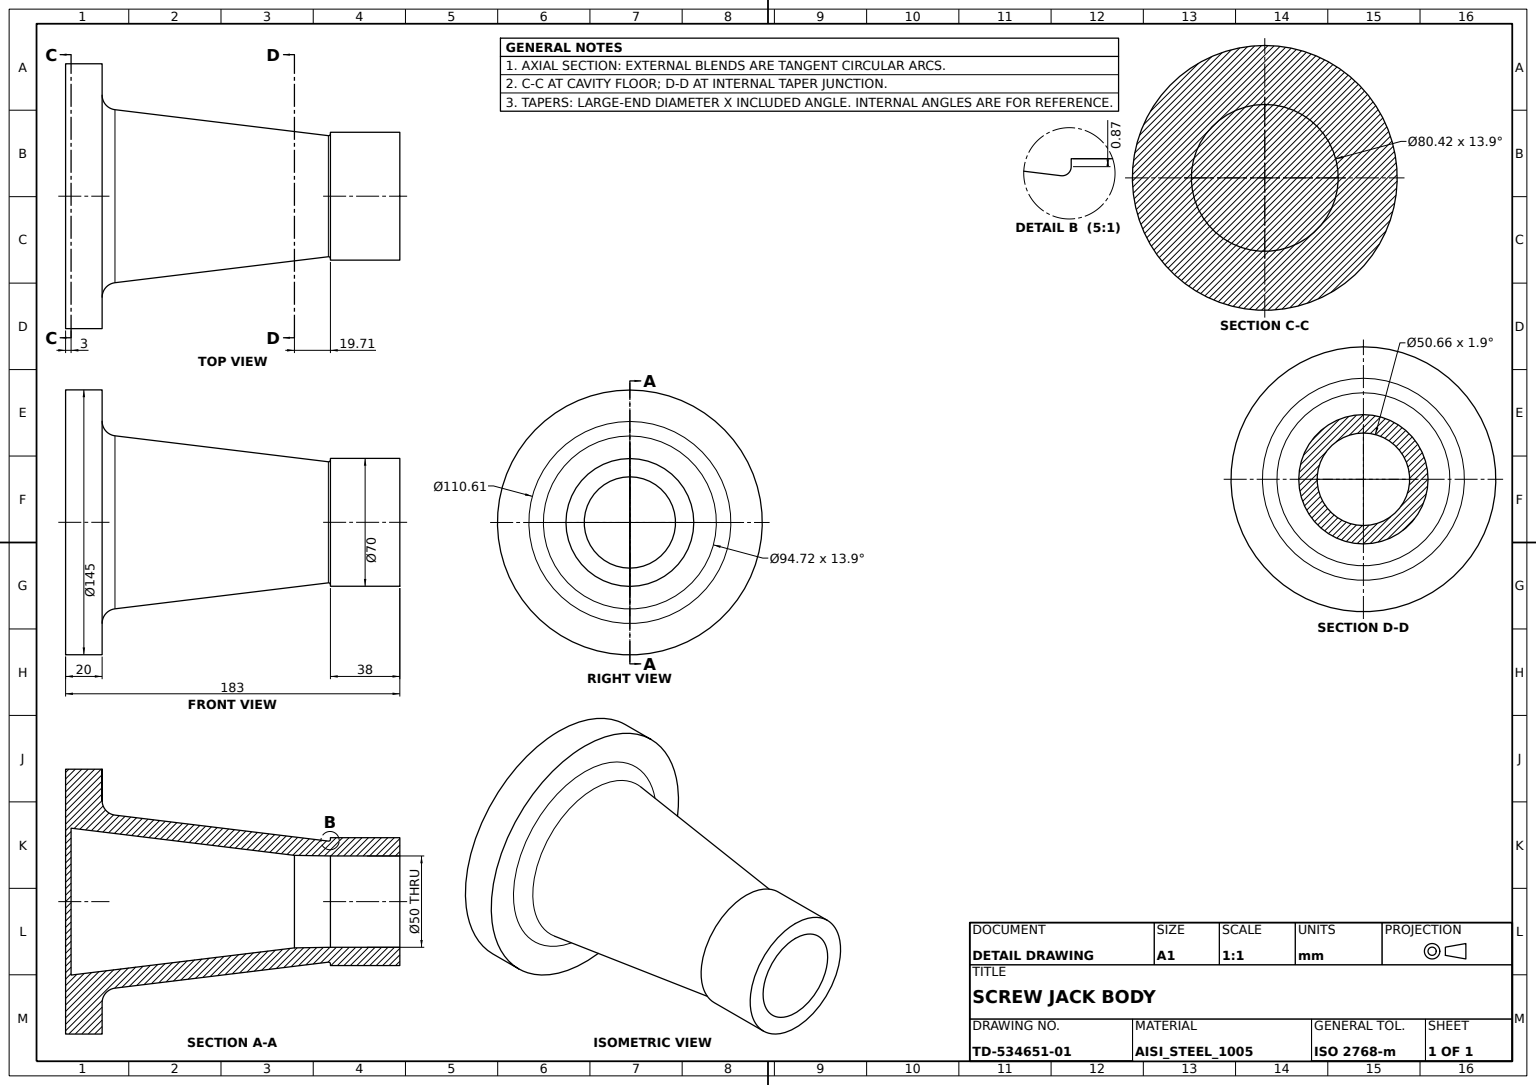
ISO-10303-21;
HEADER;
FILE_DESCRIPTION((''),'2;1');
FILE_NAME('','',(''),(''),'','','');
FILE_SCHEMA(('AUTOMOTIVE_DESIGN'));
ENDSEC;
DATA;
#1=APPLICATION_CONTEXT('');
#2=PRODUCT_CONTEXT('',#1,'mechanical');
#3=PRODUCT('','','',(#2));
#4=PRODUCT_DEFINITION_FORMATION('','',#3);
#5=PRODUCT_DEFINITION_CONTEXT('',#1,'design');
#6=PRODUCT_DEFINITION('','',#4,#5);
#7=PRODUCT_DEFINITION_SHAPE('','',#6);
#8=(LENGTH_UNIT()NAMED_UNIT(*)SI_UNIT(.MILLI.,.METRE.));
#9=(NAMED_UNIT(*)PLANE_ANGLE_UNIT()SI_UNIT($,.RADIAN.));
#10=(NAMED_UNIT(*)SI_UNIT($,.STERADIAN.)SOLID_ANGLE_UNIT());
#11=UNCERTAINTY_MEASURE_WITH_UNIT(LENGTH_MEASURE(0.005),#8,'distance_accuracy_value','');
#12=(GEOMETRIC_REPRESENTATION_CONTEXT(3)GLOBAL_UNCERTAINTY_ASSIGNED_CONTEXT((#11))GLOBAL_UNIT_ASSIGNED_CONTEXT((#8,#9,#10))REPRESENTATION_CONTEXT('',''));
#13=CARTESIAN_POINT('',(-35.,0.,183.));
#14=VERTEX_POINT('',#13);
#15=CARTESIAN_POINT('',(0.,0.,183.));
#16=DIRECTION('',(0.,0.,-1.));
#17=DIRECTION('',(-1.,0.,0.));
#18=AXIS2_PLACEMENT_3D('',#15,#16,#17);
#19=CIRCLE('',#18,35.);
#20=EDGE_CURVE('',#14,#14,#19,.T.);
#21=ORIENTED_EDGE('',*,*,#20,.F.);
#22=EDGE_LOOP('',(#21));
#23=FACE_BOUND('',#22,.T.);
#24=CARTESIAN_POINT('',(-25.,0.,183.));
#25=VERTEX_POINT('',#24);
#26=CIRCLE('',#18,25.);
#27=EDGE_CURVE('',#25,#25,#26,.T.);
#28=ORIENTED_EDGE('',*,*,#27,.T.);
#29=EDGE_LOOP('',(#28));
#30=FACE_BOUND('',#29,.T.);
#31=AXIS2_PLACEMENT_3D('',#24,#16,#17);
#32=PLANE('',#31);
#33=ADVANCED_FACE('',(#23,#30),#32,.F.);
#34=CARTESIAN_POINT('',(-33.136466,0.,143.879141));
#35=VERTEX_POINT('',#34);
#36=CARTESIAN_POINT('',(0.,0.,143.879141));
#37=AXIS2_PLACEMENT_3D('',#36,#16,#17);
#38=CIRCLE('',#37,33.136466);
#39=EDGE_CURVE('',#35,#35,#38,.T.);
#40=ORIENTED_EDGE('',*,*,#39,.F.);
#41=EDGE_LOOP('',(#40));
#42=FACE_BOUND('',#41,.T.);
#43=CARTESIAN_POINT('',(-34.129136,0.,145.));
#44=VERTEX_POINT('',#43);
#45=CARTESIAN_POINT('',(0.,0.,145.));
#46=AXIS2_PLACEMENT_3D('',#45,#16,#17);
#47=CIRCLE('',#46,34.129136);
#48=EDGE_CURVE('',#44,#44,#47,.T.);
#49=ORIENTED_EDGE('',*,*,#48,.T.);
#50=EDGE_LOOP('',(#49));
#51=FACE_BOUND('',#50,.T.);
#52=CARTESIAN_POINT('',(0.,0.,144.));
#53=AXIS2_PLACEMENT_3D('',#52,#16,#17);
#54=TOROIDAL_SURFACE('',#53,34.129136,1.);
#55=ADVANCED_FACE('',(#42,#51),#54,.F.);
#56=ORIENTED_EDGE('',*,*,#27,.F.);
#57=EDGE_LOOP('',(#56));
#58=FACE_BOUND('',#57,.T.);
#59=CARTESIAN_POINT('',(-25.,0.,145.));
#60=VERTEX_POINT('',#59);
#61=CIRCLE('',#46,25.);
#62=EDGE_CURVE('',#60,#60,#61,.T.);
#63=ORIENTED_EDGE('',*,*,#62,.T.);
#64=EDGE_LOOP('',(#63));
#65=FACE_BOUND('',#64,.T.);
#66=CARTESIAN_POINT('',(0.,0.,0.));
#67=AXIS2_PLACEMENT_3D('',#66,#16,#17);
#68=CYLINDRICAL_SURFACE('',#67,25.);
#69=ADVANCED_FACE('',(#58,#65),#68,.F.);
#70=CARTESIAN_POINT('',(-72.5,0.,0.));
#71=VERTEX_POINT('',#70);
#72=CIRCLE('',#67,72.5);
#73=EDGE_CURVE('',#71,#71,#72,.T.);
#74=ORIENTED_EDGE('',*,*,#73,.F.);
#75=EDGE_LOOP('',(#74));
#76=FACE_BOUND('',#75,.T.);
#77=CARTESIAN_POINT('',(-72.5,0.,20.));
#78=VERTEX_POINT('',#77);
#79=CARTESIAN_POINT('',(0.,0.,20.));
#80=AXIS2_PLACEMENT_3D('',#79,#16,#17);
#81=CIRCLE('',#80,72.5);
#82=EDGE_CURVE('',#78,#78,#81,.T.);
#83=ORIENTED_EDGE('',*,*,#82,.T.);
#84=EDGE_LOOP('',(#83));
#85=FACE_BOUND('',#84,.T.);
#86=CYLINDRICAL_SURFACE('',#67,72.5);
#87=ADVANCED_FACE('',(#76,#85),#86,.T.);
#88=CARTESIAN_POINT('',(-55.304009,0.,20.));
#89=VERTEX_POINT('',#88);
#90=CIRCLE('',#80,55.304009);
#91=EDGE_CURVE('',#89,#89,#90,.T.);
#92=ORIENTED_EDGE('',*,*,#91,.F.);
#93=EDGE_LOOP('',(#92));
#94=FACE_BOUND('',#93,.T.);
#95=CARTESIAN_POINT('',(-47.362651,0.,27.033127));
#96=VERTEX_POINT('',#95);
#97=CARTESIAN_POINT('',(0.,0.,27.033127));
#98=AXIS2_PLACEMENT_3D('',#97,#16,#17);
#99=CIRCLE('',#98,47.362651);
#100=EDGE_CURVE('',#96,#96,#99,.T.);
#101=ORIENTED_EDGE('',*,*,#100,.T.);
#102=EDGE_LOOP('',(#101));
#103=FACE_BOUND('',#102,.T.);
#104=CARTESIAN_POINT('',(0.,0.,28.));
#105=AXIS2_PLACEMENT_3D('',#104,#16,#17);
#106=TOROIDAL_SURFACE('',#105,55.304009,8.);
#107=ADVANCED_FACE('',(#94,#103),#106,.F.);
#108=ORIENTED_EDGE('',*,*,#62,.F.);
#109=EDGE_LOOP('',(#108));
#110=FACE_BOUND('',#109,.T.);
#111=CARTESIAN_POINT('',(-25.32582,0.,125.290481));
#112=VERTEX_POINT('',#111);
#113=CARTESIAN_POINT('',(0.,0.,125.290481));
#114=AXIS2_PLACEMENT_3D('',#113,#16,#17);
#115=CIRCLE('',#114,25.32582);
#116=EDGE_CURVE('',#112,#112,#115,.T.);
#117=ORIENTED_EDGE('',*,*,#116,.T.);
#118=EDGE_LOOP('',(#117));
#119=FACE_BOUND('',#118,.T.);
#120=CONICAL_SURFACE('',#114,25.325820168,0.016529602);
#121=ADVANCED_FACE('',(#110,#119),#120,.F.);
#122=ORIENTED_EDGE('',*,*,#82,.F.);
#123=EDGE_LOOP('',(#122));
#124=FACE_BOUND('',#123,.T.);
#125=ORIENTED_EDGE('',*,*,#91,.T.);
#126=EDGE_LOOP('',(#125));
#127=FACE_BOUND('',#126,.T.);
#128=AXIS2_PLACEMENT_3D('',#88,#16,#17);
#129=PLANE('',#128);
#130=ADVANCED_FACE('',(#124,#127),#129,.F.);
#131=CARTESIAN_POINT('',(-35.,0.,145.));
#132=VERTEX_POINT('',#131);
#133=CIRCLE('',#46,35.);
#134=EDGE_CURVE('',#132,#132,#133,.T.);
#135=ORIENTED_EDGE('',*,*,#134,.T.);
#136=EDGE_LOOP('',(#135));
#137=FACE_BOUND('',#136,.T.);
#138=ORIENTED_EDGE('',*,*,#48,.F.);
#139=EDGE_LOOP('',(#138));
#140=FACE_BOUND('',#139,.T.);
#141=DIRECTION('',(0.,0.,1.));
#142=DIRECTION('',(1.,0.,0.));
#143=AXIS2_PLACEMENT_3D('',#131,#141,#142);
#144=PLANE('',#143);
#145=ADVANCED_FACE('',(#137,#140),#144,.F.);
#146=CARTESIAN_POINT('',(-40.214878,0.,3.));
#147=VERTEX_POINT('',#146);
#148=CARTESIAN_POINT('',(0.,0.,3.));
#149=AXIS2_PLACEMENT_3D('',#148,#16,#17);
#150=CIRCLE('',#149,40.214878);
#151=EDGE_CURVE('',#147,#147,#150,.T.);
#152=ORIENTED_EDGE('',*,*,#151,.F.);
#153=EDGE_LOOP('',(#152));
#154=FACE_BOUND('',#153,.T.);
#155=PLANE('',#149);
#156=ADVANCED_FACE('',(#154),#155,.F.);
#157=ORIENTED_EDGE('',*,*,#134,.F.);
#158=EDGE_LOOP('',(#157));
#159=FACE_BOUND('',#158,.T.);
#160=ORIENTED_EDGE('',*,*,#20,.T.);
#161=EDGE_LOOP('',(#160));
#162=FACE_BOUND('',#161,.T.);
#163=CYLINDRICAL_SURFACE('',#67,35.);
#164=ADVANCED_FACE('',(#159,#162),#163,.T.);
#165=ORIENTED_EDGE('',*,*,#73,.T.);
#166=EDGE_LOOP('',(#165));
#167=FACE_BOUND('',#166,.T.);
#168=AXIS2_PLACEMENT_3D('',#70,#141,#142);
#169=PLANE('',#168);
#170=ADVANCED_FACE('',(#167),#169,.F.);
#171=ORIENTED_EDGE('',*,*,#100,.F.);
#172=EDGE_LOOP('',(#171));
#173=FACE_BOUND('',#172,.T.);
#174=ORIENTED_EDGE('',*,*,#39,.T.);
#175=EDGE_LOOP('',(#174));
#176=FACE_BOUND('',#175,.T.);
#177=CONICAL_SURFACE('',#37,33.136466348,0.121155267);
#178=ADVANCED_FACE('',(#173,#176),#177,.T.);
#179=ORIENTED_EDGE('',*,*,#151,.T.);
#180=EDGE_LOOP('',(#179));
#181=FACE_BOUND('',#180,.T.);
#182=ORIENTED_EDGE('',*,*,#116,.F.);
#183=EDGE_LOOP('',(#182));
#184=FACE_BOUND('',#183,.T.);
#185=CONICAL_SURFACE('',#149,40.214877699,0.121155267);
#186=ADVANCED_FACE('',(#181,#184),#185,.F.);
#187=CLOSED_SHELL('',(#33,#55,#69,#87,#107,#121,#130,#145,#156,#164,#170,#178,#186));
#188=MANIFOLD_SOLID_BREP('',#187);
#189=ADVANCED_BREP_SHAPE_REPRESENTATION('',(#188),#12);
#190=SHAPE_DEFINITION_REPRESENTATION(#7,#189);
ENDSEC;
END-ISO-10303-21;
